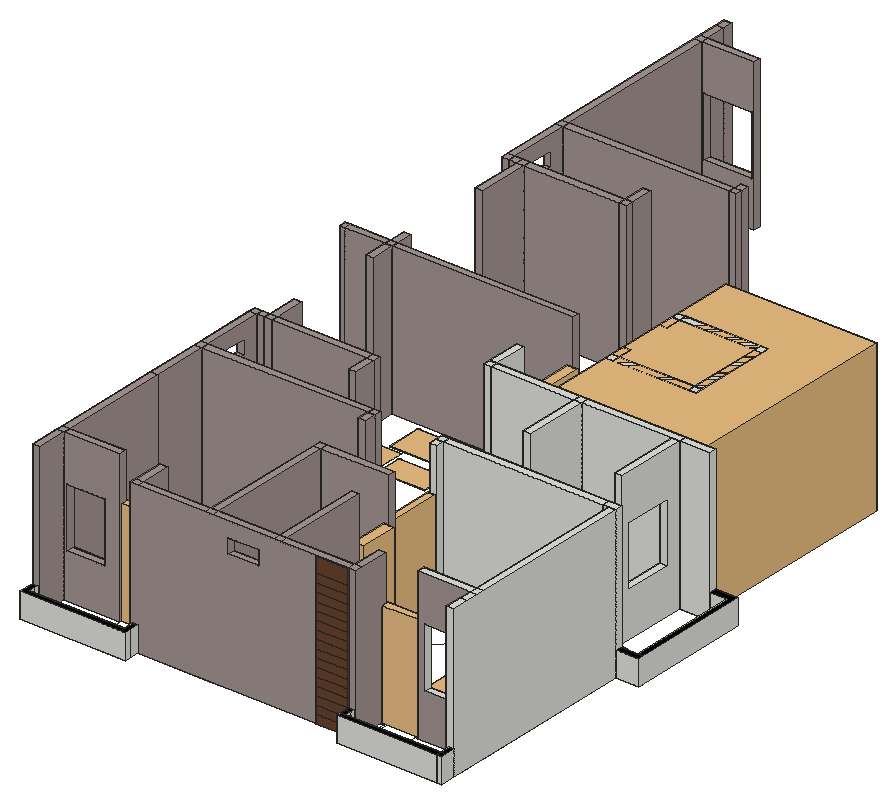
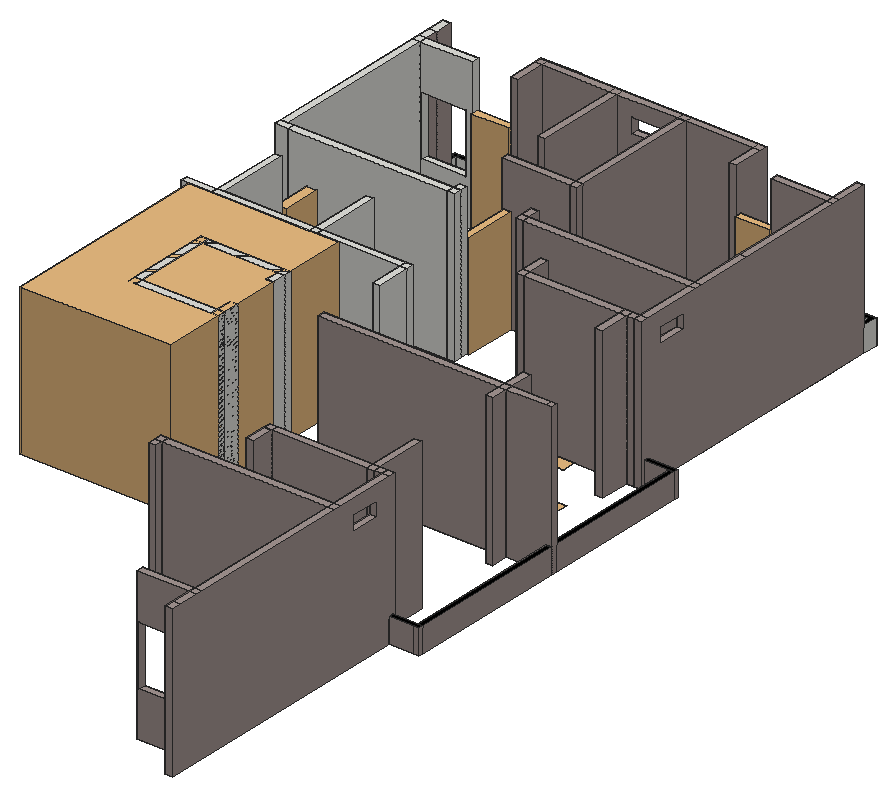
# SketchUp Ruby script. Lengths in inches.
U = 1.inch
M = Sketchup.active_model
def pt(a) = Geom::Point3d.new(a.map { |v| v * U })
def face(e, loops, mat)
  f = e.add_face(loops[0].map { |a| pt(a) })
  loops[1..].each { |l| e.add_face(l.map { |a| pt(a) }).erase! }
  f.material = f.back_material = mat if mat
  f
end
# faces: each face lists its corners as indices into pts; further lists are holes
def faces(e, pts, list, mat = nil) = list.each { |f| face(e, (f[0].is_a?(Array) ? f : [f]).map { |l| l.map { |i| pts[i] } }, mat) }
# xy, xz, yz: faces in a plane at the given z, y or x. An outline is a flat list of corners, or four numbers for a rectangle; further outlines are holes
def ring(l) = l.size == 4 ? [[l[0], l[1]], [l[2], l[1]], [l[2], l[3]], [l[0], l[3]]] : l.each_slice(2).to_a
def flat(e, list, mat, &to3) = list.each { |f| face(e, (f[0].is_a?(Array) ? f : [f]).map { |l| ring(l).map { |u, v| to3.(u, v) } }, mat) }
def xy(e, z, list, mat = nil) = flat(e, list, mat) { |x, y| [x, y, z] }
def xz(e, y, list, mat = nil) = flat(e, list, mat) { |x, z| [x, y, z] }
def yz(e, x, list, mat = nil) = flat(e, list, mat) { |y, z| [x, y, z] }
def lines(e, pts, list) = list.each { |a, b| e.add_line(pt(pts[a]), pt(pts[b])) }
# prism: a flat outline (further loops are holes) pulled along v
def prism(e, loops, v, mat = nil)
  f = face(e, loops, mat); d = Geom::Vector3d.new(v.map { |x| x * U })
  f.pushpull(f.normal.samedirection?(d) ? d.length : -d.length)
end
def box(e, o, s, mat = nil) = prism(e, [[o, [o[0] + s[0], o[1], o[2]], [o[0] + s[0], o[1] + s[1], o[2]], [o[0], o[1] + s[1], o[2]]]], [0, 0, s[2]], mat)
def at(x, y, z, deg = 0) = Geom::Transformation.translation(pt([x, y, z])) * Geom::Transformation.rotation(ORIGIN, Z_AXIS, deg.degrees)
def axes(o, x, y, z) = Geom::Transformation.new([*x, 0, *y, 0, *z, 0, *pt(o).to_a, 1])
def part(name) = M.definitions.add(name)
# library, detail: a bought-in or finely detailed component or shape, given as its bounding box
def library(name, o, s) = part(name).tap { |d| box(d.entities, o, s) }
def detail(e, o, s) = box(e.add_group.entities, o, s)
def put(e, d, t, mat = nil) = e.add_instance(d, t).tap { |i| i.material = mat if mat }
def group(e, t, mat = nil) = e.add_group.tap { |g| g.transformation = t; g.material = mat if mat }.entities
root = M.entities
M.materials.add("M09_Shadow_Night").color = [0, 0, 0]
M.materials.add("Marble_06_1K").color = [165, 150, 147]
M.materials.add("Wood_Veneer_15_1K").color = [103, 69, 45]
c1 = part("Group\#8")
xy(c1.entities,0,[[0,-8.88,4,-4.88],[4,-8.88,80,-4.88],[80,-8.88,84,-4.88],[0,-4.88,4,0],[80,-4.88,84,3.12],
  [0,0,4,3.12]])
xy(c1.entities,20,[[0,-8.88,4,-4.88],[4,-8.88,80,-4.88],[80,-8.88,84,-4.88],[0,-4.88,4,0],[80,-4.88,84,3.12],
  [0,0,4,3.12]],"M09_Shadow_Night")
xz(c1.entities,-8.88,[[0,0,80,20],[80,0,84,20]])
xz(c1.entities,-4.88,[[4,0,80,20]])
xz(c1.entities,3.12,[[0,0,4,20],[80,0,84,20]])
yz(c1.entities,0,[[-8.88,0,3.12,20]])
yz(c1.entities,4,[[-4.88,0,0,20],[0,0,3.12,20]])
yz(c1.entities,80,[[-8.88,0,-4.88,20],[-4.88,0,3.12,20]])
yz(c1.entities,84,[[-8.88,0,3.12,20]])
c2 = part("Group\#6")
xy(c2.entities,0,[[0,-8,80,-4],[80,-8,84,-4],[0,-4,4,0],[80,-4,84,4],[0,0,4,4]])
xy(c2.entities,20,[[0,-8,84,-8,84,4,80,4,80,-4,4,-4,4,4,0,4]],"M09_Shadow_Night")
xz(c2.entities,-8,[[0,0,84,20]])
xz(c2.entities,-4,[[4,0,80,20]])
xz(c2.entities,4,[[0,0,4,20],[80,0,84,20]])
yz(c2.entities,0,[[-8,0,4,20]])
yz(c2.entities,4,[[-4,0,0,20],[0,0,4,20]])
yz(c2.entities,80,[[-4,0,4,20]])
yz(c2.entities,84,[[-8,0,-4,20],[-4,0,4,20]])
c3 = library("TREE-26",[-60.96,-72.91,0],[121.92,134.74,0.01])
c4 = part("Group\#116")
xy(c4.entities,0,[[24,0,24.75,24.75]])
xy(c4.entities,107,[[24,0,24.75,24.75]])
xz(c4.entities,0,[[24,0,24.75,107]])
xz(c4.entities,24.75,[[24,0,24.75,107]])
yz(c4.entities,24,[[0,0,24.75,6],[0,6,24.75,12],[0,12,24.75,18],[0,18,24.75,24],[0,24,24.75,30],
  [0,30,24.75,36],[0,36,24.75,42],[0,42,24.75,48],[0,48,24.75,54],[0,54,24.75,60],
  [0,60,24.75,66],[0,66,24.75,72],[0,72,24.75,78],[0,78,24.75,84],[0,84,24.75,90],
  [0,90,24.75,96],[0,96,24.75,107]],"Wood_Veneer_15_1K")
yz(c4.entities,24.75,[[0,0,24.75,107]])
c5 = part("tgr")
p = [[-2.37,-3.35,0],[-2.37,-2.82,0],[-2.73,-2.82,0],[-2.73,-2.68,0],[-3.71,-2.68,0],[-3.71,-3.35,0],
  [-2.37,3.35,0],[-2.37,2.82,0],[-2.73,2.82,0],[-2.73,2.68,0],[-3.71,2.68,0],[-3.71,3.35,0],
  [3.71,-2.82,0],[-2.37,-2.46,0],[3.71,-2.46,0],[3.7,-2.46,0],[3.63,-2.07,0],[3.53,-1.68,0],
  [3.41,-1.3,0],[3.27,-0.93,0],[3.1,-0.57,0],[2.91,-0.22,0],[2.7,0.12,0],[2.46,0.4375,0],
  [2.21,0.74,0],[1.93,1.03,0],[1.64,1.3,0],[1.33,1.55,0],[1.01,1.79,0],[0.67,1.99,0],
  [0.32,2.18,0],[-0.04,2.35,0],[-0.41,2.49,0],[-0.8,2.6,0],[-1.18,2.69,0],[-1.58,2.76,0],
  [-1.97,2.8,0]]
lines(c5.entities,p,[[0,1],[1,2],[2,3],[3,4],[4,5],[5,0],[6,7],[7,8],[8,9],[9,10],[10,11],[11,6],
  [1,12],[13,14],[1,13],[12,14],[15,16],[16,17],[17,18],[18,19],[19,20],[20,21],[21,22],[22,23],
  [23,24],[24,25],[25,26],[26,27],[27,28],[28,29],[29,30],[30,31],[31,32],[32,33],[33,34],[34,35],
  [35,36],[36,7]])
c6 = library("Component\#2",[1075.72,38.58,0],[54,24,0.01])
c7 = library("Component\#1",[961.32,38.58,0],[54,24,0.01])
c8 = library("ghgjg",[-265.23,-341.01,0],[530.46,682.02,0.01])
c9 = library("Group\#51",[0,0,0],[6.9375,42,86.5])
c10 = part("GTGTGYHYHYHY")
p = [[-3.29,3.76,0],[3.29,3.76,0],[3.29,-3.76,0],[-3.29,-3.76,0]]
lines(c10.entities,p,[[0,1],[1,2],[2,3],[3,0],[0,2],[1,3]])
c11 = part("G5GTGTGT")
p = [[0.52,4.97,0],[0.52,-4.97,0],[0.36,-4.97,0],[0.36,4.97,0],[-0.08,-4.53,0],[-0.08,4.53,0],
  [0.33,4.97,0],[0.3,4.97,0],[0.28,4.96,0],[0.25,4.96,0],[0.22,4.95,0],[0.2,4.94,0],
  [0.17,4.93,0],[0.15,4.92,0],[0.12,4.9,0],[0.1,4.89,0],[0.08,4.87,0],[0.06,4.85,0],
  [0.04,4.83,0],[0.02,4.8125,0],[0,4.79,0],[-0.01,4.77,0],[-0.03,4.74,0],[-0.04,4.72,0],
  [-0.05,4.69,0],[-0.0625,4.67,0],[-0.07,4.64,0],[-0.08,4.61,0],[-0.08,4.59,0],[-0.08,4.56,0],
  [-0.08,-4.56,0],[-0.08,-4.59,0],[-0.08,-4.61,0],[-0.07,-4.64,0],[-0.0625,-4.67,0],[-0.05,-4.69,0],
  [-0.04,-4.72,0],[-0.03,-4.74,0],[-0.01,-4.77,0],[0,-4.79,0],[0.02,-4.8125,0],[0.04,-4.83,0],
  [0.06,-4.85,0],[0.08,-4.87,0],[0.1,-4.89,0],[0.12,-4.9,0],[0.15,-4.92,0],[0.17,-4.93,0],
  [0.2,-4.94,0],[0.22,-4.95,0],[0.25,-4.96,0],[0.28,-4.96,0],[0.3,-4.97,0],[0.33,-4.97,0],
  [-0.08,-1.38,0],[-0.52,-1.38,0],[-0.08,1.38,0],[-0.52,1.38,0]]
lines(c11.entities,p,[[0,1],[1,2],[2,3],[3,0],[4,5],[3,6],[6,7],[7,8],[8,9],[9,10],[10,11],[11,12],
  [12,13],[13,14],[14,15],[15,16],[16,17],[17,18],[18,19],[19,20],[20,21],[21,22],[22,23],[23,24],
  [24,25],[25,26],[26,27],[27,28],[28,29],[29,5],[4,30],[30,31],[31,32],[32,33],[33,34],[34,35],
  [35,36],[36,37],[37,38],[38,39],[39,40],[40,41],[41,42],[42,43],[43,44],[44,45],[45,46],[46,47],
  [47,48],[48,49],[49,50],[50,51],[51,52],[52,53],[53,2],[54,55],[56,57],[55,57]])
c12 = library("lcd-01",[-577.99,-134.75,0],[1155.98,269.5,0.01])
c13 = library("Group\#49",[0,0,0],[8.31,30,84])
c14 = library("JEEW",[-211.14,-299.86,0],[422.28,599.72,0.01])
c15 = library("double bed",[-999.9375,-1062.5,0],[1999.875,2125,0.01])
c16 = part("EGWF")
p = [[2.59,-3.49,0],[2.59,-3.09,0],[2.85,-3.09,0],[2.85,-2.99,0],[3.58,-2.99,0],[3.58,-3.49,0],
  [2.59,3.49,0],[2.59,3.09,0],[2.85,3.09,0],[2.85,2.99,0],[3.58,2.99,0],[3.58,3.49,0],
  [-3.58,-3.09,0],[2.59,-2.82,0],[-3.58,-2.82,0],[2.2,3.07,0],[1.81,3.04,0],[1.42,2.97,0],
  [1.03,2.89,0],[0.66,2.78,0],[0.29,2.64,0],[-0.07,2.48,0],[-0.42,2.3,0],[-0.76,2.1,0],
  [-1.08,1.875,0],[-1.39,1.63,0],[-1.68,1.37,0],[-1.96,1.09,0],[-2.21,0.79,0],[-2.45,0.48,0],
  [-2.67,0.15,0],[-2.86,-0.1875,0],[-3.04,-0.54,0],[-3.1875,-0.9,0],[-3.32,-1.28,0],[-3.42,-1.66,0],
  [-3.5,-2.04,0],[-3.55,-2.43,0]]
lines(c16.entities,p,[[0,1],[1,2],[2,3],[3,4],[4,5],[5,0],[6,7],[7,8],[8,9],[9,10],[10,11],[11,6],
  [1,12],[13,14],[1,13],[12,14],[7,15],[15,16],[16,17],[17,18],[18,19],[19,20],[20,21],[21,22],
  [22,23],[23,24],[24,25],[25,26],[26,27],[27,28],[28,29],[29,30],[30,31],[31,32],[32,33],[33,34],
  [34,35],[35,36],[36,37],[37,14]])
c17 = library("Group\#50",[0,0,0],[6.9375,42,86.5])
c18 = part("Group\#10")
xy(c18.entities,0,[[-133.3,-6,-127.3,0],[-133.3,0,-127.3,6],[-127.3,0,0,6],[0,0,10.7,6]])
xy(c18.entities,120,[[-133.3,-6,-127.3,0],[-133.3,0,-127.3,6],[-127.3,0,0,6],[0,0,10.7,6]])
xz(c18.entities,-6,[[-133.3,0,-127.3,120]])
xz(c18.entities,0,[[-133.3,0,-127.3,120],[-127.3,0,0,120],[0,0,10.7,120]])
xz(c18.entities,6,[[-133.3,0,-127.3,120],[-127.3,0,0,120],[0,0,10.7,120]])
yz(c18.entities,-133.3,[[-6,0,0,120],[0,0,6,120]])
yz(c18.entities,-127.3,[[-6,0,0,120],[0,0,6,120]])
yz(c18.entities,0,[[0,0,6,120]])
yz(c18.entities,10.7,[[0,0,6,120]])
c19 = library("A$C72E23588",[-1177.7,-903.95,0],[2355.4,1807.9,0.01])
c20 = part("Group\#11")
xy(c20.entities,0,[[0,0,5.15,4],[5.15,0,13.95,4],[13.95,0,18,4],[13.95,4,18,93],[-30,36,-24,93],
  [-108,42,-102,93],[-180.4,93,-174.4,99],[-174.4,93,-108,99],[-108,93,-102,99],[-102,93,-24,99],
  [-24,93,-6,99],[-6,93,0,99],[0,93,13.95,99],[13.95,93,18,99],[-180.4,99,-174.4,126.21]])
xy(c20.entities,20,[[0,0,18,4],[13.95,4,18,4,18,99,0,99,0,93,13.95,93]],"M09_Shadow_Night")
xy(c20.entities,36,[[-30,42,-24,81]])
xy(c20.entities,84,[[-30,42,-24,81]])
xy(c20.entities,120,[[-30,36,-24,93],[-108,42,-102,93],[-180.4,93,-174.4,99],[-174.4,93,-108,99],[-108,93,-102,99],
  [-102,93,-24,99],[-24,93,0,99],[-180.4,99,-174.4,126.21]])
xz(c20.entities,0,[[0,0,18,20]])
xz(c20.entities,4,[[0,0,5.15,20],[5.15,0,13.95,20]])
xz(c20.entities,36,[[-30,0,-24,120]])
xz(c20.entities,42,[[-108,0,-102,120],[-30,36,-24,84]])
xz(c20.entities,81,[[-30,36,-24,84]])
xz(c20.entities,93,[[-180.4,0,-174.4,120],[-174.4,0,-108,120],[-108,0,-102,120],[-102,0,-30,120],[-30,0,-24,120],
  [-24,0,0,120],[0,0,13.95,20]])
xz(c20.entities,99,[[-180.4,0,-174.4,120],[-174.4,0,-108,120],[-108,0,-102,120],[-102,0,-24,120],[-24,0,-6,120],
  [-6,0,0,120],[0,0,18,20]])
xz(c20.entities,126.21,[[-180.4,0,-174.4,120]])
yz(c20.entities,-180.4,[[93,0,99,120],[99,0,126.21,120]])
yz(c20.entities,-174.4,[[93,0,99,120],[99,0,126.21,120]])
yz(c20.entities,-108,[[42,0,93,120],[93,0,99,120]])
yz(c20.entities,-102,[[42,0,93,120],[93,0,99,120]])
yz(c20.entities,-30,[[[36,0,93,120],[42,36,81,84]]])
yz(c20.entities,-24,[[[36,0,93,120],[42,36,81,84]],[93,0,99,120]])
yz(c20.entities,0,[[0,0,4,20],[93,0,99,20],[93,20,99,120]])
yz(c20.entities,13.95,[[4,0,93,20]])
yz(c20.entities,18,[[0,0,99,20]])
c21 = library("BFGFV",[-4.32,-2.51,0],[8.64,5.02,0.01])
c22 = library("VVVV",[-3.39,-3.68,0],[6.78,7.36,0.01])
c23 = part("feeeeeeeeee")
p = [[-2.68,3.51,0],[-2.68,3.16,0],[-2.92,3.16,0],[-2.92,3.07,0],[-3.56,3.07,0],[-3.56,3.51,0],
  [-2.68,-3.51,0],[-2.68,-3.16,0],[-2.92,-3.16,0],[-2.92,-3.07,0],[-3.56,-3.07,0],[-3.56,-3.51,0],
  [3.56,3.16,0],[-2.68,2.93,0],[3.56,2.93,0],[-2.48,-3.13,0],[-2.04,-3.07,0],[-1.61,-2.98,0],
  [-1.1875,-2.86,0],[-0.77,-2.72,0],[-0.36,-2.55,0],[0.03,-2.35,0],[0.41,-2.13,0],[0.78,-1.88,0],
  [1.125,-1.62,0],[1.46,-1.32,0],[1.77,-1.01,0],[2.06,-0.68,0],[2.33,-0.33,0],[2.57,0.03,0],
  [2.79,0.42,0],[2.99,0.81,0],[3.16,1.22,0],[3.3,1.63,0],[3.41,2.06,0],[3.5,2.49,0]]
lines(c23.entities,p,[[0,1],[1,2],[2,3],[3,4],[4,5],[5,0],[6,7],[7,8],[8,9],[9,10],[10,11],[11,6],
  [1,12],[13,14],[1,13],[12,14],[8,15],[15,16],[16,17],[17,18],[18,19],[19,20],[20,21],[21,22],
  [22,23],[23,24],[24,25],[25,26],[26,27],[27,28],[28,29],[29,30],[30,31],[31,32],[32,33],[33,34],
  [34,35],[35,14]])
c24 = library("HYHHYHYHYHYHY",[-2.09,-4.54,0],[4.18,9.08,0.01])
c25 = part("Group\#53")
xy(c25.entities,0,[[-66,-66,-60,-60],[-60,-66,0,-60],[0,-66,6,-60],[-66,-60,-60,-48.73],[0,-60,6,0],
  [-66,-12.73,-60,0],[-66,0,-60,6],[-60,0,0,6],[0,0,6,6]])
xy(c25.entities,120,[[-66,-66,-60,-60],[-60,-66,0,-60],[0,-66,6,-60],[-66,-60,-60,-48.73],[0,-60,6,0],
  [-66,-12.73,-60,0],[-66,0,-60,6],[-60,0,0,6],[0,0,6,6]])
xz(c25.entities,-66,[[-66,0,-60,120],[-60,0,0,120],[0,0,6,120]])
xz(c25.entities,-60,[[-66,0,-60,120],[-60,0,0,120],[0,0,6,120]])
xz(c25.entities,-48.73,[[-66,0,-60,120]])
xz(c25.entities,-12.73,[[-66,0,-60,120]])
xz(c25.entities,0,[[-66,0,-60,120],[-60,0,0,120],[0,0,6,120]])
xz(c25.entities,6,[[-66,0,-60,120],[-60,0,0,120],[0,0,6,120]])
yz(c25.entities,-66,[[-66,0,-60,120],[-60,0,-48.73,120],[-12.73,0,0,120],[0,0,6,120]])
yz(c25.entities,-60,[[-66,0,-60,120],[-60,0,-48.73,120],[-12.73,0,0,120],[0,0,6,120]])
yz(c25.entities,0,[[-66,0,-60,120],[-60,0,0,120],[0,0,6,120]])
yz(c25.entities,6,[[-66,0,-60,120],[-60,0,0,120],[0,0,6,120]])
c26 = library("Return staircase",[0,-11.89,0],[120,168,120])
xy(root,372,[[109.8,55.34,163.8,79.34],[224.2,55.34,278.2,79.1]])
put(root,c1,at(278.2,46.22,372))
put(root,c2,at(25.8,45.34,372))
put(root,c3,axes([36.72,48.3,372],[0,0.1317,0],[0.1317,0,0],[0,0,0.1317]),"Marble_06_1K")
put(root,c3,axes([350.625,48.65,372],[0,0.1317,0],[0.1317,0,0],[0,0,0.1317]),"Marble_06_1K")
put(root,c4,axes([278.2,24.59,372],[0,1,0],[-1.02586,0,0],[0,0,1.1215]),"Wood_Veneer_15_1K")
put(root,c5,axes([299.2,62.74,372],[0,-4.47464,0],[4.47464,0,0],[0,0,4.47464]),"Marble_06_1K")
put(root,c5,axes([88.8,62.74,372],[0,-4.47464,0],[-4.47464,0,0],[0,0,4.47464]),"Marble_06_1K")
put(root,c6,at(-851.52,16.76,372),"Marble_06_1K")
put(root,c7,at(-851.52,16.76,372),"Marble_06_1K")
put(root,c8,axes([194,68.98,372],[0.04,0,0],[0,-0.04,0],[0,0,0.04]),"Marble_06_1K")
put(root,c9,axes([284.2,81,372],[0,-0.85622,0],[0.71429,0,0],[0,0,0.9711]))
put(root,c9,axes([76.2,81,372],[0,-0.85622,0],[0.65714,0,0],[0,0,0.9711]))
put(root,c10,axes([330.2,104.34,372],[0,-2.12603,0],[2.12603,0,0],[0,0,2.12603]),"Marble_06_1K")
g1 = group(root,at(103.8,49.34,372),"Marble_06_1K")
xy(g1,0,[[0,0,6,6],[6,0,60,6],[60,0,66,6],[66,0,114.4,6],[114.4,0,120.4,6],
  [120.4,0,174.4,6],[174.4,0,180.4,6],[0,6,6,30],[60,6,66,108],[114.4,6,120.4,78],
  [174.4,6,180.4,30],[60,108,66,114],[66,108,120.4,114]])
xy(g1,96,[[78,0,102.4,6]])
xy(g1,108,[[78,0,102.4,6]])
xy(g1,120,[[0,0,6,6],[6,0,60,6],[60,0,66,6],[66,0,114.4,6],[114.4,0,120.4,6],
  [120.4,0,174.4,6],[174.4,0,180.4,6],[0,6,6,30],[60,6,66,108],[114.4,6,120.4,78],
  [174.4,6,180.4,30],[60,108,66,114],[66,108,120.4,114]])
xz(g1,0,[[[0,0,180.4,120],[78,96,102.4,108]]])
xz(g1,6,[[6,0,60,120],[60,0,66,120],[[66,0,114.4,120],[78,96,102.4,108]],[114.4,0,120.4,120],[120.4,0,174.4,120]])
xz(g1,30,[[0,0,6,120],[174.4,0,180.4,120]])
xz(g1,78,[[114.4,0,120.4,120]])
xz(g1,108,[[60,0,66,120],[66,0,120.4,120]])
xz(g1,114,[[60,0,66,120],[66,0,120.4,120]])
yz(g1,0,[[0,0,30,120]])
yz(g1,6,[[6,0,30,120]])
yz(g1,60,[[6,0,108,120],[108,0,114,120]])
yz(g1,66,[[6,0,108,120],[108,0,114,120]])
yz(g1,78,[[0,96,6,108]])
yz(g1,102.4,[[0,96,6,108]])
yz(g1,114.4,[[6,0,78,120]])
yz(g1,120.4,[[6,0,78,120],[108,0,114,120]])
yz(g1,174.4,[[6,0,30,120]])
yz(g1,180.4,[[0,0,30,120]])
# 1 loose lines left out
put(root,c11,axes([226.1,107.57,372],[3.62,0,0],[0,3.62,0],[0,0,3.62]),"Marble_06_1K")
put(root,c12,axes([158.41,128.75,372],[0,-0.04,0],[0.04,0,0],[0,0,0.04]),"Marble_06_1K")
g2 = group(root,at(356.2,49.34,372))
xy(g2,0,[[0,0,6,13.86],[0,13.86,6,24],[-42,24,0,30],[0,24,6,30],[0,30,6,162]])
xy(g2,36,[[-36,24,-1,30]])
xy(g2,84,[[-36,24,-1,30]])
xy(g2,120,[[0,0,6,13.86],[0,13.86,6,24],[-42,24,0,30],[0,24,6,30],[0,30,6,162]])
xz(g2,0,[[0,0,6,120]])
xz(g2,24,[[[-42,0,0,120],[-36,36,-1,84]]],"Marble_06_1K")
xz(g2,30,[[[-42,0,0,120],[-36,36,-1,84]]])
xz(g2,162,[[0,0,6,120]])
yz(g2,-42,[[24,0,30,120]])
yz(g2,-36,[[24,36,30,84]])
yz(g2,-1,[[24,36,30,84]])
yz(g2,0,[[24,0,30,120],[30,0,162,120]])
yz(g2,0,[[0,0,13.86,120],[13.86,0,24,120]],"Marble_06_1K")
yz(g2,6,[[0,0,162,120]])
put(root,c5,axes([207.6,142.34,372],[-4.47464,0,0],[0,-4.47464,0],[0,0,4.47464]),"Marble_06_1K")
put(root,c13,at(219.92,127.34,372))
put(root,c14,axes([178.84,144.49,372],[-0.04284,0,0],[0,0.04284,0],[0,0,0.04284]),"Marble_06_1K")
put(root,c15,axes([316.9375,148.2,372],[0,-0.03695,0],[0.03695,0,0],[0,0,0.03695]),"Marble_06_1K")
put(root,c15,axes([71.06,148.29,372],[0,-0.03695,0],[-0.03695,0,0],[0,0,0.03695]),"Marble_06_1K")
put(root,c13,axes([163.72,163.34,372],[1,0,0],[0,1.28434,0],[0,0,1]))
put(root,c16,axes([148.2,184.34,372],[6.02515,0,0],[0,-6.02515,0],[0,0,6.02515]),"Marble_06_1K")
put(root,c17,axes([216.54,163.34,372],[0.85622,0,0],[0,1,0],[0,0,0.9711]))
put(root,c16,axes([239.8,184.34,372],[-6.02515,0,0],[0,-6.02515,0],[0,0,6.02515]),"Marble_06_1K")
put(root,c18,at(351.5,211.34,372))
put(root,c3,axes([371.8,222.26,372],[0,0.1317,0],[0.1317,0,0],[0,0,0.1317]),"Marble_06_1K")
put(root,c13,axes([336.48,247.16,372],[-1,0,0],[0,-0.994,0],[0,0,1]))
put(root,c5,axes([109.2,232.34,372],[-4.47464,0,0],[0,4.47464,0],[0,0,4.47464]),"Marble_06_1K")
put(root,c9,axes([127.46,247.34,372],[-0.85622,0,0],[0,-0.71429,0],[0,0,0.9711]))
put(root,c5,axes([348.8,232.34,372],[4.47464,0,0],[0,4.47464,0],[0,0,4.47464]),"Marble_06_1K")
put(root,c8,axes([45.4375,241.34,372],[0,-0.04,0],[-0.04,0,0],[0,0,0.04]),"Marble_06_1K")
put(root,c14,axes([106.95,256.29,372],[0,0.04284,0],[0.04284,0,0],[0,0,0.04284]),"Marble_06_1K")
put(root,c19,axes([191.83,263.52,372],[0.0356,0,0],[0,-0.0356,0],[0,0,0.0356]),"Marble_06_1K")
put(root,c20,at(362.2,211.34,372))
put(root,c3,axes([12.58,274.84,372],[0,0.1317,0],[0.1317,0,0],[0,0,0.1317]),"Marble_06_1K")
put(root,c12,axes([102.68,276.73,372],[0.04,0,0],[0,-0.04,0],[0,0,0.04]),"Marble_06_1K")
put(root,c3,axes([371.8,298.64,372],[0,0.1317,0],[0.1317,0,0],[0,0,0.1317]),"Marble_06_1K")
put(root,c21,axes([101.4,333.38,372],[4.3395,0,0],[0,-4.3395,0],[0,0,4.3395]),"Marble_06_1K")
put(root,c22,axes([64.42,333.77,372],[4.47564,0,0],[0,-4.47564,0],[0,0,4.47564]),"Marble_06_1K")
put(root,c22,axes([138,333.77,372],[-4.47564,0,0],[0,-4.47564,0],[0,0,4.47564]),"Marble_06_1K")
put(root,c23,axes([163.46,361.55,372],[-6.83664,0,0],[0,6.83664,0],[0,0,6.83664]),"Marble_06_1K")
put(root,c13,axes([183.52,337.55,372],[1,0,0],[0,1.6118,0],[0,0,1]))
put(root,c24,axes([99.08,366.86,372],[0,6.75189,0],[6.75189,0,0],[0,0,6.75189]),"Marble_06_1K")
put(root,c3,axes([12.58,379.27,372],[0,0.1317,0],[0.1317,0,0],[0,0,0.1317]),"Marble_06_1K")
g3 = group(root,at(25.8,731.54,372),"Marble_06_1K")
xy(g3,0,[[12,-255.51,18,-214.2],[0,-214.2,6,-208.2],[6,-214.2,12,-208.2],[12,-214.2,18,-208.2],[18,-214.2,94,-208.2],
  [94,-214.2,100,-208.2],[0,-208.2,6,-160.2],[94,-208.2,100,-190.2],[0,-160.2,6,-154.2],[6,-160.2,138,-154.2],
  [138,-160.2,144,-154.2],[0,-154.2,6,-116.77],[138,-154.2,144,-148.2],[0,-116.77,6,-80.17],[0,-80.17,6,-22.2],
  [0,-22.2,6,-16.2],[6,-22.2,48,-16.2],[0,-16.2,6,0],[0,0,6,7.73]])
xy(g3,36,[[8,-22.2,46,-16.2]])
xy(g3,84,[[8,-22.2,46,-16.2]])
xy(g3,96,[[0,-196.2,6,-172.2]])
xy(g3,108,[[0,-196.2,6,-172.2]])
xy(g3,120,[[12,-255.51,18,-214.2],[0,-214.2,6,-208.2],[6,-214.2,12,-208.2],[12,-214.2,18,-208.2],[18,-214.2,94,-208.2],
  [94,-214.2,100,-208.2],[0,-208.2,6,-160.2],[94,-208.2,100,-190.2],[0,-160.2,6,-154.2],[6,-160.2,138,-154.2],
  [138,-160.2,144,-154.2],[0,-154.2,6,-22.2],[138,-154.2,144,-148.2],[0,-22.2,6,-16.2],[6,-22.2,48,-16.2],
  [0,-16.2,6,0],[0,0,6,7.73]])
xz(g3,-255.51,[[12,0,18,120]])
xz(g3,-214.2,[[0,0,6,120],[6,0,12,120],[12,0,18,120],[18,0,94,120],[94,0,100,120]])
xz(g3,-208.2,[[6,0,12,120],[12,0,18,120],[18,0,94,120],[94,0,100,120]])
xz(g3,-196.2,[[0,96,6,108]])
xz(g3,-190.2,[[94,0,100,120]])
xz(g3,-172.2,[[0,96,6,108]])
xz(g3,-160.2,[[6,0,138,120],[138,0,144,120]])
xz(g3,-154.2,[[6,0,138,120],[138,0,144,120]])
xz(g3,-148.2,[[138,0,144,120]])
xz(g3,-22.2,[[[6,0,48,120],[8,36,46,84]]])
xz(g3,-16.2,[[[6,0,48,120],[8,36,46,84]]])
xz(g3,7.73,[[0,0,6,120]])
yz(g3,0,[[[-214.2,0,7.73,120],[-196.2,96,-172.2,108]]])
yz(g3,6,[[-214.2,0,-208.2,120],[[-208.2,0,-160.2,120],[-196.2,96,-172.2,108]],[-160.2,0,-154.2,120],[-154.2,0,-22.2,120],[-22.2,0,-16.2,120],
  [-16.2,0,0,120],[0,0,7.73,120]])
yz(g3,8,[[-22.2,36,-16.2,84]])
yz(g3,12,[[-214.2,0,-208.2,120]])
yz(g3,12,[[-255.51,0,-214.2,120]],"Marble_06_1K")
yz(g3,18,[[-255.51,0,-214.2,120],[-214.2,0,-208.2,120]])
yz(g3,46,[[-22.2,36,-16.2,84]])
yz(g3,48,[[-22.2,0,-16.2,120]])
yz(g3,94,[[-214.2,0,-208.2,120],[-208.2,0,-190.2,120]])
yz(g3,100,[[-214.2,0,-208.2,120],[-208.2,0,-190.2,120]])
yz(g3,138,[[-160.2,0,-154.2,120],[-154.2,0,-148.2,120]])
yz(g3,144,[[-160.2,0,-154.2,120],[-154.2,0,-148.2,120]])
g4 = group(g3,at(-2.625,-212.2,0))
xy(g4,0,[[2.625,-470,8.625,-446],[2.625,-446,8.625,-440],[8.625,-446,53.03,-440],[2.625,-440,8.625,-352.75],[2.625,-352.75,8.625,-308],
  [140.625,-317.47,146.625,-308],[2.625,-308,8.625,-302],[8.625,-308,140.625,-302],[140.625,-308,146.625,-302],[2.625,-302,8.625,-254],
  [96.625,-272,102.625,-254],[-21.375,-254,-17.27,-250],[-17.27,-254,2.625,-250],[2.625,-254,8.625,-250],[8.625,-254,14.625,-250],
  [14.625,-254,20.625,-250],[20.625,-254,96.625,-250],[96.625,-254,102.625,-250],[-21.375,-250,-17.27,-133.43],[2.625,-250,8.625,-248],
  [8.625,-250,14.625,-248],[14.625,-250,20.625,-248],[20.625,-250,96.625,-248],[96.625,-250,102.625,-248],[14.625,-248,20.625,-224],
  [14.625,-152,20.625,-133.43],[-21.375,-133.43,-17.27,-127.79],[-17.27,-133.43,14.625,-127.79],[14.625,-133.43,20.625,-127.79],[20.625,-133.43,164.625,-127.79],
  [-21.375,-127.79,-17.27,0],[14.625,-127.79,20.625,-114.45],[-21.375,0,-17.27,4],[-17.27,0,2.625,4]])
xy(g4,20,[[-21.375,-254,2.625,-250],[-21.375,-250,-17.27,-133.43],[-21.375,-127.79,-17.27,0],[-21.375,0,2.625,4]],"M09_Shadow_Night")
xy(g4,36,[[11.33,-446,41.03,-440]])
xy(g4,84,[[11.33,-446,41.03,-440]])
xy(g4,96,[[2.625,-290,8.625,-266]])
xy(g4,108,[[2.625,-290,8.625,-266]])
xy(g4,119.9375,[[96.625,-272,102.625,-254]])
xy(g4,120,[[2.625,-470,8.625,-446],[2.625,-446,8.625,-440],[8.625,-446,53.03,-440],[2.625,-440,8.625,-352.75],[2.625,-352.75,8.625,-308],
  [140.625,-317.47,146.625,-308],[2.625,-308,8.625,-302],[8.625,-308,140.625,-302],[140.625,-308,146.625,-302],[2.625,-302,8.625,-254],
  [2.625,-254,8.625,-248],[8.625,-254,14.625,-248],[14.625,-254,20.625,-248],[20.625,-254,96.625,-248],[96.625,-254,102.625,-248],
  [14.625,-248,20.625,-224],[14.625,-152,20.625,-133.43],[-21.375,-133.43,-17.27,-127.79],[-17.27,-133.43,14.625,-127.79],[14.625,-133.43,20.625,-127.79],
  [20.625,-133.43,164.625,-127.79],[14.625,-127.79,20.625,-114.45]])
xz(g4,-470,[[2.625,0,8.625,120]])
xz(g4,-446,[[[8.625,0,53.03,120],[11.33,36,41.03,84]]],"Marble_06_1K")
xz(g4,-440,[[[8.625,0,53.03,120],[11.33,36,41.03,84]]])
xz(g4,-317.47,[[140.625,0,146.625,120]])
xz(g4,-308,[[8.625,0,140.625,120],[140.625,0,146.625,120]])
xz(g4,-302,[[8.625,0,140.625,120],[140.625,0,146.625,120]])
xz(g4,-290,[[2.625,96,8.625,108]])
xz(g4,-272,[[96.625,0,102.625,119.9375]])
xz(g4,-266,[[2.625,96,8.625,108]])
xz(g4,-254,[[-21.375,0,-17.27,20],[-17.27,0,2.625,20],[8.625,0,14.625,120],[14.625,0,20.625,120],[20.625,0,96.625,120],
  [96.625,0,102.625,119.9375],[96.625,119.9375,102.625,120]])
xz(g4,-250,[[-21.375,0,-17.27,20],[-17.27,0,2.625,20]])
xz(g4,-248,[[14.625,0,20.625,120],[20.625,0,96.625,120],[96.625,0,102.625,120]])
xz(g4,-248,[[2.625,0,8.625,120],[8.625,0,14.625,120]],"Marble_06_1K")
xz(g4,-224,[[14.625,0,20.625,120]])
xz(g4,-152,[[14.625,0,20.625,120]])
xz(g4,-133.43,[[-21.375,0,-17.27,20],[14.625,0,20.625,120],[20.625,0,164.625,120],[-21.375,20,-17.27,120]])
xz(g4,-133.43,[[-17.27,0,14.625,120]],"Marble_06_1K")
xz(g4,-127.79,[[-21.375,0,-17.27,20],[14.625,0,20.625,120],[20.625,0,164.625,120]])
xz(g4,-127.79,[[-17.27,0,-17.27,20,-21.375,20,-21.375,120,14.625,120,14.625,0]],"Marble_06_1K")
xz(g4,-114.45,[[14.625,0,20.625,120]])
xz(g4,0,[[-21.375,0,-17.27,20],[-17.27,0,2.625,20]])
xz(g4,4,[[-21.375,0,-17.27,20],[-17.27,0,2.625,20]])
yz(g4,-21.375,[[-254,0,-250,20],[-250,0,-133.43,20],[-133.43,0,-127.79,120],[-127.79,0,0,20],[0,0,4,20]])
yz(g4,-17.27,[[-250,0,-133.43,20],[-127.79,0,0,20]])
yz(g4,2.625,[[[-470,0,-470,120,-248,120,-248,0,-250,0,-250,20,-254,20,-254,0],[-290,96,-266,108]],[-254,0,-250,20],[0,0,4,20]])
yz(g4,8.625,[[-446,0,-440,120],[-440,0,-352.75,120],[-352.75,0,-308,120],[-308,0,-302,120],[[-302,0,-254,120],[-290,96,-266,108]],
  [-254,0,-248,120]])
yz(g4,8.625,[[-470,0,-446,120]],"Marble_06_1K")
yz(g4,11.33,[[-446,36,-440,84]])
yz(g4,14.625,[[-254,0,-248,120],[-133.43,0,-127.79,120]])
yz(g4,14.625,[[-248,0,-224,120],[-152,0,-133.43,120],[-127.79,0,-114.45,120]],"Marble_06_1K")
yz(g4,20.625,[[-254,0,-248,120],[-248,0,-224,120],[-152,0,-133.43,120],[-133.43,0,-127.79,120],[-127.79,0,-114.45,120]])
yz(g4,41.03,[[-446,36,-440,84]])
yz(g4,53.03,[[-446,0,-440,120]])
yz(g4,96.625,[[-272,0,-254,119.9375],[-254,0,-248,120]])
yz(g4,102.625,[[-272,0,-254,119.9375],[-254,0,-248,120]])
yz(g4,140.625,[[-317.47,0,-308,120],[-308,0,-302,120]])
yz(g4,146.625,[[-317.47,0,-308,120],[-308,0,-302,120]])
yz(g4,164.625,[[-133.43,0,-127.79,120]])
put(root,c25,at(302.2,424.34,372))
put(root,c26,at(236.2,322.23,372))
